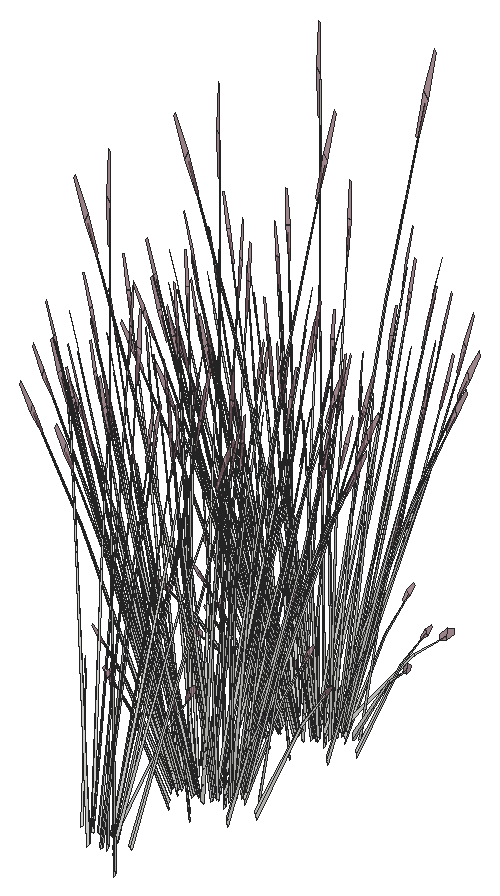
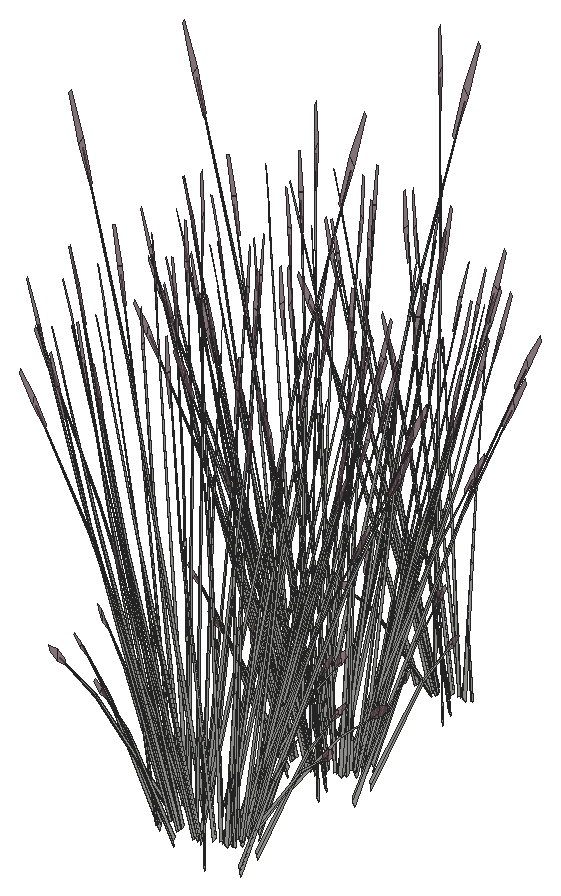
# SketchUp Ruby script. Lengths in inches.
U = 1.inch
M = Sketchup.active_model
def pt(a) = Geom::Point3d.new(a.map { |v| v * U })
def face(e, loops, mat)
  f = e.add_face(loops[0].map { |a| pt(a) })
  loops[1..].each { |l| e.add_face(l.map { |a| pt(a) }).erase! }
  f.material = f.back_material = mat if mat
  f
end
# faces: each face lists its corners as indices into pts; further lists are holes
def faces(e, pts, list, mat = nil) = list.each { |f| face(e, (f[0].is_a?(Array) ? f : [f]).map { |l| l.map { |i| pts[i] } }, mat) }
# xy, xz, yz: faces in a plane at the given z, y or x. An outline is a flat list of corners, or four numbers for a rectangle; further outlines are holes
def ring(l) = l.size == 4 ? [[l[0], l[1]], [l[2], l[1]], [l[2], l[3]], [l[0], l[3]]] : l.each_slice(2).to_a
def flat(e, list, mat, &to3) = list.each { |f| face(e, (f[0].is_a?(Array) ? f : [f]).map { |l| ring(l).map { |u, v| to3.(u, v) } }, mat) }
def xy(e, z, list, mat = nil) = flat(e, list, mat) { |x, y| [x, y, z] }
def xz(e, y, list, mat = nil) = flat(e, list, mat) { |x, z| [x, y, z] }
def yz(e, x, list, mat = nil) = flat(e, list, mat) { |y, z| [x, y, z] }
def lines(e, pts, list) = list.each { |a, b| e.add_line(pt(pts[a]), pt(pts[b])) }
# prism: a flat outline (further loops are holes) pulled along v
def prism(e, loops, v, mat = nil)
  f = face(e, loops, mat); d = Geom::Vector3d.new(v.map { |x| x * U })
  f.pushpull(f.normal.samedirection?(d) ? d.length : -d.length)
end
def box(e, o, s, mat = nil) = prism(e, [[o, [o[0] + s[0], o[1], o[2]], [o[0] + s[0], o[1] + s[1], o[2]], [o[0], o[1] + s[1], o[2]]]], [0, 0, s[2]], mat)
def at(x, y, z, deg = 0) = Geom::Transformation.translation(pt([x, y, z])) * Geom::Transformation.rotation(ORIGIN, Z_AXIS, deg.degrees)
def axes(o, x, y, z) = Geom::Transformation.new([*x, 0, *y, 0, *z, 0, *pt(o).to_a, 1])
def part(name) = M.definitions.add(name)
# library, detail: a bought-in or finely detailed component or shape, given as its bounding box
def library(name, o, s) = part(name).tap { |d| box(d.entities, o, s) }
def detail(e, o, s) = box(e.add_group.entities, o, s)
def put(e, d, t, mat = nil) = e.add_instance(d, t).tap { |i| i.material = mat if mat }
def group(e, t, mat = nil) = e.add_group.tap { |g| g.transformation = t; g.material = mat if mat }.entities
root = M.entities
M.materials.add("LightPink_Translucent").color = [144, 107, 117]
M.materials["LightPink_Translucent"].alpha = 0.75
c1 = part("blade")
p = [[2.15,0.21,22],[0,0.17,0],[0.09,0.45,0],[2.18,0.31,22],[2.29,0.31,22],[0.38,0.45,0],
  [2.48,0.24,33],[2.49,0.24,33],[2.48,0.22,33]]
faces(c1.entities,p,[[0,1,2,3],[4,5,2,3],[6,3,4,7],[8,0,3,6]])
c2 = part("seeds")
p = [[0.3,-0.1,1.38],[-0.01,-0.03,1.59],[-0.01,-0.03,0.03],[0.14,-0.07,-0.07],[0.29,-0.03,3],[0.15,0.01,3.11]]
faces(c2.entities,p,[[0,1,2,3],[1,0,4,5]],"LightPink_Translucent")
c3 = part("blade with seeds")
put(c3.entities,c1,at(0,0,0))
put(c3.entities,c2,axes([2.4,0.25,30.99],[1.5799,-0.05474,1.17369],[-0.12525,1.92788,0.29478],[-0.07173,-0.02425,1.56792]))
put(root,c3,axes([334.74,315.96,50.51],[-0.01379,-0.36791,1.24828],[0.62424,0.09537,0.52853],[-0.14764,0.20132,1.17828]))
put(root,c3,axes([334.79,317.375,52.14],[0.49824,-0.09289,-0.45151],[0.08716,0.35177,-0.34973],[0.13382,0.10081,0.86392]))
put(root,c3,axes([332.16,316.625,51.43],[0.09401,-0.13431,1.51428],[0.3944,0.27795,0.12244],[-0.17792,0.17323,0.64734]))
put(root,c3,axes([332.27,317.38,52],[-0.34164,0.20573,-0.31292],[-0.3234,-0.23491,0.40398],[-0.04921,0.11936,0.77298]))
put(root,c3,axes([331.09,317.32,52.17],[-0.01255,0.07733,1.54581],[0.35618,0.269,-0.24447],[-0.09325,0.12721,0.12397]))
put(root,c3,axes([333.25,317.55,52.45],[0.49409,-0.18193,-0.10745],[0.24281,0.32289,-0.59638],[0.06519,0.13607,0.90619]))
put(root,c3,axes([332.48,318.18,50.44],[-0.01307,-0.23234,1.01491],[0.32652,0.16572,0.74569],[-0.06422,0.11074,0.22354]))
put(root,c3,axes([332.61,317.28,52.42],[0.36145,0.26255,-0.50118],[-0.38183,0.22994,-0.3882],[-0.055,0.1334,0.95895]))
put(root,c3,axes([333.68,317.54,52.14],[0.49634,0.09796,-0.45151],[-0.17013,0.33585,-0.34973],[0.04551,0.13522,0.86392]))
put(root,c3,axes([333.96,316.85,51.43],[-0.11542,-0.12546,1.51428],[0.53333,-0.10562,0.12244],[0.12054,0.19696,0.64734]))
put(root,c3,axes([333.45,317.74,52],[-0.15222,0.30049,-0.31292],[-0.44409,-0.08764,0.40398],[0.04072,0.12098,0.77298]))
put(root,c3,axes([332.49,317.16,52.72],[-0.01314,0.36145,-0.69681],[-0.55324,-0.02428,0.08409],[-0.05838,0.15313,0.9857]))
put(root,c3,axes([333.02,316.91,51.43],[-0.01236,-0.14998,1.51428],[0.53562,0.09949,0.12244],[-0.03313,0.21373,0.64734]))
put(root,c3,axes([333.5,317.47,52.4],[0.24099,0.31773,-0.62776],[-0.49607,0.17707,0.07576],[0.05635,0.15352,0.88802]))
put(root,c3,axes([333.14,318.28,52.17],[0.064,0.06292,1.54581],[0.51651,0.02472,-0.24447],[0.05194,0.13877,0.12397]))
put(root,c3,axes([332.31,317.67,50.97],[0.01109,-0.20172,1.3638],[0.49896,0.10655,0.18846],[-0.04323,0.21498,0.64398]))
put(root,c3,axes([332.69,324.99,51.43],[0.11542,0.12546,1.51428],[-0.53333,0.10562,0.12244],[-0.12054,-0.19696,0.64734]))
put(root,c3,axes([334.11,325.08,52.4],[-0.24099,-0.31773,-0.62776],[0.49607,-0.17707,0.07576],[-0.05635,-0.15352,0.88802]))
put(root,c3,axes([335.12,325.39,52.4],[0.01314,-0.36145,-0.62776],[0.55324,0.02428,0.07576],[0.05838,-0.15313,0.88802]))
put(root,c3,axes([334.16,324.81,52],[0.15222,-0.30049,-0.31292],[0.44409,0.08764,0.40398],[-0.04072,-0.12098,0.77298]))
put(root,c3,axes([334.5,325.21,51.43],[-0.09401,0.13431,1.51428],[-0.3944,-0.27795,0.12244],[0.17792,-0.17323,0.64734]))
put(root,c3,axes([333.93,325.02,52.14],[-0.49634,-0.09796,-0.45151],[0.17013,-0.33585,-0.34973],[-0.04551,-0.13522,0.86392]))
put(root,c3,axes([334.24,324.18,50.44],[0.06477,0.22786,1.01491],[-0.35932,-0.1262,0.74569],[0.03867,-0.11667,0.22354]))
put(root,c3,axes([335.01,325.27,52.14],[-0.36145,-0.26255,-0.45151],[0.38183,-0.22994,-0.34973],[0.055,-0.1334,0.86392]))
put(root,c3,axes([334.36,325,52.45],[-0.49409,0.18193,-0.10745],[-0.24281,-0.32289,-0.59638],[-0.06519,-0.13607,0.90619]))
put(root,c3,axes([335.38,325.41,52.45],[-0.55492,-0.01936,-0.10745],[0.01517,-0.36657,-0.59638],[0.03855,-0.14118,0.90619]))
put(root,c3,axes([335.35,325.17,52],[0.34164,-0.20573,-0.31292],[0.3234,0.23491,0.40398],[0.04921,-0.11936,0.77298]))
put(root,c3,axes([332.39,324.45,50.44],[0.26338,0.136,1.01491],[-0.38358,0.08175,0.74569],[-0.08207,-0.10452,0.22354]))
put(root,c3,axes([333.03,325.17,52.4],[-0.43054,-0.18887,-0.62776],[0.30598,-0.33097,0.07576],[-0.15599,-0.11277,0.88802]))
put(root,c3,axes([332.88,324.92,52],[-0.07798,-0.31474,-0.31292],[0.44579,-0.08311,0.40398],[-0.11974,-0.09019,0.77298]))
put(root,c3,axes([331.92,325.38,51.43],[0.18755,0.06732,1.51428],[-0.38813,0.28243,0.12244],[-0.24191,-0.12741,0.64734]))
put(root,c3,axes([332.83,325.18,52.14],[-0.49824,0.09289,-0.45151],[-0.08716,-0.35177,-0.34973],[-0.13382,-0.10081,0.86392]))
put(root,c3,axes([335.77,326.02,52.4],[0.26374,-0.30832,-0.62776],[0.46217,0.21911,0.07576],[0.15748,-0.11171,0.88802]))
put(root,c3,axes([335.76,325.875,52.14],[-0.12971,-0.3568,-0.45151],[0.49122,-0.06241,-0.34973],[0.14077,-0.09583,0.86392]))
put(root,c3,axes([335.99,326.13,52.45],[-0.46706,-0.21546,-0.10745],[0.26908,-0.31203,-0.59638],[0.13196,-0.10846,0.90619]))
put(root,c3,axes([334.06,327.31,50.9375],[0.43633,0.15757,1.33654],[-0.42745,0.33945,0.52853],[-0.19146,-0.20119,1.12046]))
put(root,c3,axes([336.36,325.17,50.44],[-0.16818,0.19891,1.01491],[-0.14456,-0.26725,0.74569],[0.1389,-0.06697,0.22354]))
put(root,c3,axes([336.12,325.91,52],[0.43951,-0.05584,-0.31292],[0.11606,0.31924,0.40398],[0.12595,-0.08575,0.77298]))
put(root,c3,axes([331.85,325.47,52],[-0.28729,-0.24465,-0.31292],[0.32804,-0.23159,0.40398],[-0.16667,-0.03524,0.77298]))
put(root,c3,axes([332.15,325.64,52.4],[-0.50473,-0.00941,-0.62776],[0.0339,-0.39618,0.07576],[-0.21383,-0.04181,0.88802]))
put(root,c3,axes([331.98,325.72,52.14],[-0.36663,0.25884,-0.45151],[-0.32109,-0.27343,-0.34973],[-0.18628,-0.03938,0.86392]))
put(root,c3,axes([331.16,326.0625,50.44],[0.32236,-0.02796,1.01491],[-0.20448,0.24636,0.74569],[-0.1593,-0.03696,0.22354]))
put(root,c3,axes([332.18,325.45,52.45],[-0.02704,0.39739,-0.10745],[-0.51189,-0.01086,-0.59638],[-0.19715,-0.0276,0.90619]))
put(root,c3,axes([336.01,326.97,52.45],[-0.25405,-0.35383,-0.10745],[0.45089,-0.17388,-0.59638],[0.19001,-0.04668,0.90619]))
put(root,c3,axes([335.98,326.67,52.14],[0.13679,-0.35544,-0.45151],[0.46898,0.12183,-0.34973],[0.18882,-0.03259,0.86392]))
put(root,c3,axes([331.52,325.99,51.43],[0.20943,-0.00885,1.51428],[-0.13893,0.38357,0.12244],[-0.29846,-0.02372,0.64734]))
put(root,c3,axes([335.9,326.8,52.4],[0.44368,-0.17257,-0.62776],[0.24726,0.35524,0.07576],[0.21437,-0.04035,0.88802]))
put(root,c3,axes([336.27,326.83,52],[0.41962,0.10901,-0.31292],[-0.12239,0.31802,0.40398],[0.16894,-0.02916,0.77298]))
put(root,c3,axes([331.34,326.32,52],[-0.41962,-0.10901,-0.31292],[0.12239,-0.31802,0.40398],[-0.16894,0.02916,0.77298]))
put(root,c3,axes([335.13,326.4375,51.43],[-0.20943,0.00885,1.51428],[0.13893,-0.38357,0.12244],[0.29846,0.02372,0.64734]))
put(root,c3,axes([332.62,326.27,50.95],[0.14352,-0.05653,1.56454],[0.04949,0.39467,0.12244],[-0.31087,0.05237,0.55918]))
put(root,c3,axes([337.16,326.89,50.44],[-0.31197,0.06451,1.01491],[0.14684,-0.26661,0.74569],[0.1655,0.01824,0.22354]))
put(root,c3,axes([331.63,326.49,52.14],[-0.13679,0.35544,-0.45151],[-0.46898,-0.12183,-0.34973],[-0.18882,0.03259,0.86392]))
put(root,c3,axes([331.61,326.18,52.45],[0.25405,0.35383,-0.10745],[-0.45089,0.17388,-0.59638],[-0.19001,0.04668,0.90619]))
put(root,c3,axes([336.62,327.72,51.47],[-0.09664,-0.32847,-0.03085],[0.45676,-0.07551,-0.13989],[0.09538,0.02082,0.4614]))
put(root,c3,axes([335.4375,327.71,52.45],[0.02704,-0.39739,-0.10745],[0.51189,0.01086,-0.59638],[0.19715,0.0276,0.90619]))
put(root,c3,axes([331.61,326.67,51.43],[0.17519,-0.08265,1.51428],[0.14749,0.38193,0.12244],[-0.27504,0.08632,0.64734]))
put(root,c3,axes([335.46,327.52,52.4],[0.50473,0.00941,-0.62776],[-0.0339,0.39618,0.07576],[0.21383,0.04181,0.88802]))
put(root,c3,axes([330.7,328.01,50.44],[0.21042,-0.1771,1.01491],[0.08303,0.28036,0.74569],[-0.15207,0.0502,0.22354]))
put(root,c3,axes([335.77,327.68,52],[0.28729,0.24465,-0.31292],[-0.32804,0.23159,0.40398],[0.16667,0.03524,0.77298]))
put(root,c3,axes([331.49,327.24,52],[-0.43951,0.05584,-0.31292],[-0.11606,-0.31924,0.40398],[-0.12595,0.08575,0.77298]))
put(root,c3,axes([334.73,327.05,51.43],[-0.18755,-0.06732,1.51428],[0.38813,-0.28243,0.12244],[0.24191,0.12741,0.64734]))
put(root,c3,axes([334.77,326.17,51.95],[-0.4363,-0.20303,1.22187],[0.46069,-0.31611,0.5272],[0.14077,0.1905,1.18105]))
put(root,c3,axes([331.625,327.02,52.45],[0.46706,0.21546,-0.10745],[-0.26908,0.31203,-0.59638],[-0.13196,0.10846,0.90619]))
put(root,c3,axes([335.43,327.82,50.44],[-0.28429,-0.11236,1.01491],[0.36709,-0.11416,0.74569],[0.09901,0.0967,0.22354]))
put(root,c3,axes([334.43,328.14,52.45],[0.30087,-0.33447,-0.10745],[0.43572,0.19269,-0.59638],[0.15146,0.0945,0.90619]))
put(root,c3,axes([332.25,326.93,51.43],[0.12611,-0.12006,1.51428],[0.31843,0.32408,0.12244],[-0.2184,0.14759,0.64734]))
put(root,c3,axes([331.86,327.28,52.14],[0.12971,0.3568,-0.45151],[-0.49122,0.06241,-0.34973],[-0.14077,0.09583,0.86392]))
put(root,c3,axes([334.74,326.55,50.51],[-0.01379,-0.36791,1.24828],[0.62424,0.09537,0.52853],[-0.14764,0.20132,1.17828]))
put(root,c3,axes([334.79,327.97,52.14],[0.49824,-0.09289,-0.45151],[0.08716,0.35177,-0.34973],[0.13382,0.10081,0.86392]))
put(root,c3,axes([332.16,327.22,51.43],[0.09401,-0.13431,1.51428],[0.3944,0.27795,0.12244],[-0.17792,0.17323,0.64734]))
put(root,c3,axes([332.27,327.98,52],[-0.34164,0.20573,-0.31292],[-0.3234,-0.23491,0.40398],[-0.04921,0.11936,0.77298]))
put(root,c3,axes([333.25,328.15,52.45],[0.49409,-0.18193,-0.10745],[0.24281,0.32289,-0.59638],[0.06519,0.13607,0.90619]))
put(root,c3,axes([332.48,328.78,50.44],[-0.01307,-0.23234,1.01491],[0.32652,0.16572,0.74569],[-0.06422,0.11074,0.22354]))
put(root,c3,axes([332.61,327.88,52.42],[0.36145,0.26255,-0.50118],[-0.38183,0.22994,-0.3882],[-0.055,0.1334,0.95895]))
put(root,c3,axes([333.68,328.14,52.14],[0.49634,0.09796,-0.45151],[-0.17013,0.33585,-0.34973],[0.04551,0.13522,0.86392]))
put(root,c3,axes([333.96,327.44,51.43],[-0.11542,-0.12546,1.51428],[0.53333,-0.10562,0.12244],[0.12054,0.19696,0.64734]))
put(root,c3,axes([333.45,328.34,52],[-0.15222,0.30049,-0.31292],[-0.44409,-0.08764,0.40398],[0.04072,0.12098,0.77298]))
put(root,c3,axes([332.49,327.76,52.72],[-0.01314,0.36145,-0.69681],[-0.55324,-0.02428,0.08409],[-0.05838,0.15313,0.9857]))
put(root,c3,axes([333.02,327.51,51.43],[-0.01236,-0.14998,1.51428],[0.53562,0.09949,0.12244],[-0.03313,0.21373,0.64734]))
put(root,c3,axes([332.69,334.69,51.43],[0.11542,0.12546,1.51428],[-0.53333,0.10562,0.12244],[-0.12054,-0.19696,0.64734]))
put(root,c3,axes([333.5,328.07,52.4],[0.24099,0.31773,-0.62776],[-0.49607,0.17707,0.07576],[0.05635,0.15352,0.88802]))
put(root,c3,axes([333.57,333.86,52.17],[-0.07723,-0.05479,1.54581],[-0.51538,0.03473,-0.24447],[-0.08225,-0.13104,0.12397]))
put(root,c3,axes([334.11,334.78,52.4],[-0.24099,-0.31773,-0.62776],[0.49607,-0.17707,0.07576],[-0.05635,-0.15352,0.88802]))
put(root,c3,axes([335.12,335.1,52.4],[0.01314,-0.36145,-0.62776],[0.55324,0.02428,0.07576],[0.05838,-0.15313,0.88802]))
put(root,c3,axes([332.31,328.27,50.97],[0.01109,-0.20172,1.3638],[0.49896,0.10655,0.18846],[-0.04323,0.21498,0.64398]))
put(root,c3,axes([335.89,334.53,52.17],[-0.00487,-0.07777,1.54581],[-0.41166,-0.22476,-0.24447],[0.06364,-0.13625,0.12397]))
put(root,c3,axes([334.16,334.51,52],[0.15222,-0.30049,-0.31292],[0.44409,0.08764,0.40398],[-0.04072,-0.12098,0.77298]))
put(root,c3,axes([334.5,334.91,51.43],[-0.09401,0.13431,1.51428],[-0.3944,-0.27795,0.12244],[0.17792,-0.17323,0.64734]))
put(root,c3,axes([333.93,334.72,52.14],[-0.49634,-0.09796,-0.45151],[0.17013,-0.33585,-0.34973],[-0.04551,-0.13522,0.86392]))
put(root,c3,axes([334.24,333.88,50.44],[0.06477,0.22786,1.01491],[-0.35932,-0.1262,0.74569],[0.03867,-0.11667,0.22354]))
put(root,c3,axes([335.01,334.98,52.14],[-0.36145,-0.26255,-0.45151],[0.38183,-0.22994,-0.34973],[0.055,-0.1334,0.86392]))
put(root,c3,axes([334.36,334.7,52.45],[-0.49409,0.18193,-0.10745],[-0.24281,-0.32289,-0.59638],[-0.06519,-0.13607,0.90619]))
put(root,c3,axes([335.38,335.11,52.45],[-0.55492,-0.01936,-0.10745],[0.01517,-0.36657,-0.59638],[0.03855,-0.14118,0.90619]))
put(root,c3,axes([335.35,334.88,52],[0.34164,-0.20573,-0.31292],[0.3234,0.23491,0.40398],[0.04921,-0.11936,0.77298]))
put(root,c3,axes([332.39,334.15,50.44],[0.26338,0.136,1.01491],[-0.38358,0.08175,0.74569],[-0.08207,-0.10452,0.22354]))
put(root,c3,axes([333.03,334.875,52.4],[-0.43054,-0.18887,-0.62776],[0.30598,-0.33097,0.07576],[-0.15599,-0.11277,0.88802]))
put(root,c3,axes([332.88,334.625,52],[-0.07798,-0.31474,-0.31292],[0.44579,-0.08311,0.40398],[-0.11974,-0.09019,0.77298]))
put(root,c3,axes([331.92,335.08,51.43],[0.18755,0.06732,1.51428],[-0.38813,0.28243,0.12244],[-0.24191,-0.12741,0.64734]))
put(root,c3,axes([332.83,334.88,52.14],[-0.49824,0.09289,-0.45151],[-0.08716,-0.35177,-0.34973],[-0.13382,-0.10081,0.86392]))
put(root,c3,axes([335.77,335.72,52.4],[0.26374,-0.30832,-0.62776],[0.46217,0.21911,0.07576],[0.15748,-0.11171,0.88802]))
put(root,c3,axes([335.76,335.58,52.14],[-0.12971,-0.3568,-0.45151],[0.49122,-0.06241,-0.34973],[0.14077,-0.09583,0.86392]))
put(root,c3,axes([331.88,334.46,52.17],[-0.10864,-0.00276,1.54581],[-0.34587,0.27582,-0.24447],[-0.18454,-0.05636,0.12397]))
put(root,c3,axes([335.99,335.84,52.45],[-0.46706,-0.21546,-0.10745],[0.26908,-0.31203,-0.59638],[0.13196,-0.10846,0.90619]))
put(root,c3,axes([334.06,337.01,50.9375],[0.43633,0.15757,1.33654],[-0.42745,0.33945,0.52853],[-0.19146,-0.20119,1.12046]))
put(root,c3,axes([336.36,334.87,50.44],[-0.16818,0.19891,1.01491],[-0.14456,-0.26725,0.74569],[0.1389,-0.06697,0.22354]))
put(root,c3,axes([336.12,335.62,52],[0.43951,-0.05584,-0.31292],[0.11606,0.31924,0.40398],[0.12595,-0.08575,0.77298]))
put(root,c3,axes([331.85,335.18,52],[-0.28729,-0.24465,-0.31292],[0.32804,-0.23159,0.40398],[-0.16667,-0.03524,0.77298]))
put(root,c3,axes([332.15,335.34,52.4],[-0.50473,-0.00941,-0.62776],[0.0339,-0.39618,0.07576],[-0.21383,-0.04181,0.88802]))
put(root,c3,axes([337.39,336.12,52.17],[0.07006,-0.05952,1.54581],[-0.08968,-0.3651,-0.24447],[0.1758,-0.06922,0.12397]))
put(root,c3,axes([331.98,335.42,52.14],[-0.36663,0.25884,-0.45151],[-0.32109,-0.27343,-0.34973],[-0.18628,-0.03938,0.86392]))
put(root,c3,axes([331.16,335.77,50.44],[0.32236,-0.02796,1.01491],[-0.20448,0.24636,0.74569],[-0.1593,-0.03696,0.22354]))
put(root,c3,axes([332.18,335.15,52.45],[-0.02704,0.39739,-0.10745],[-0.51189,-0.01086,-0.59638],[-0.19715,-0.0276,0.90619]))
put(root,c3,axes([336.01,336.68,52.45],[-0.25405,-0.35383,-0.10745],[0.45089,-0.17388,-0.59638],[0.19001,-0.04668,0.90619]))
put(root,c3,axes([335.98,336.37,52.14],[0.13679,-0.35544,-0.45151],[0.46898,0.12183,-0.34973],[0.18882,-0.03259,0.86392]))
put(root,c3,axes([331.52,335.7,51.43],[0.20943,-0.00885,1.51428],[-0.13893,0.38357,0.12244],[-0.29846,-0.02372,0.64734]))
put(root,c3,axes([335.9,336.5,52.4],[0.44368,-0.17257,-0.62776],[0.24726,0.35524,0.07576],[0.21437,-0.04035,0.88802]))
put(root,c3,axes([336.27,336.53,52],[0.41962,0.10901,-0.31292],[-0.12239,0.31802,0.40398],[0.16894,-0.02916,0.77298]))
put(root,c3,axes([331.34,336.03,52],[-0.41962,-0.10901,-0.31292],[0.12239,-0.31802,0.40398],[-0.16894,0.02916,0.77298]))
put(root,c3,axes([335.13,336.14,51.43],[-0.20943,0.00885,1.51428],[0.13893,-0.38357,0.12244],[0.29846,0.02372,0.64734]))
put(root,c3,axes([332.62,335.97,50.95],[0.14352,-0.05653,1.56454],[0.04949,0.39467,0.12244],[-0.31087,0.05237,0.55918]))
put(root,c3,axes([337.16,336.6,50.44],[-0.31197,0.06451,1.01491],[0.14684,-0.26661,0.74569],[0.1655,0.01824,0.22354]))
put(root,c3,axes([331.08,336.24,52.17],[-0.08245,0.05073,1.54581],[0.00701,0.37067,-0.24447],[-0.18899,0.0482,0.12397]))
put(root,c3,axes([331.63,336.19,52.14],[-0.13679,0.35544,-0.45151],[-0.46898,-0.12183,-0.34973],[-0.18882,0.03259,0.86392]))
put(root,c3,axes([331.61,335.89,52.45],[0.25405,0.35383,-0.10745],[-0.45089,0.17388,-0.59638],[-0.19001,0.04668,0.90619]))
put(root,c3,axes([336.62,337.42,51.47],[-0.09664,-0.32847,-0.03085],[0.45676,-0.07551,-0.13989],[0.09538,0.02082,0.4614]))
put(root,c3,axes([335.4375,337.41,52.45],[0.02704,-0.39739,-0.10745],[0.51189,0.01086,-0.59638],[0.19715,0.0276,0.90619]))
put(root,c3,axes([335.88,337.17,52.17],[0.10831,-0.00661,1.54581],[0.29709,-0.30358,-0.24447],[0.19266,0.04007,0.12397]))
put(root,c3,axes([331.61,336.375,51.43],[0.17519,-0.08265,1.51428],[0.14749,0.38193,0.12244],[-0.27504,0.08632,0.64734]))
put(root,c3,axes([335.46,337.22,52.4],[0.50473,0.00941,-0.62776],[-0.0339,0.39618,0.07576],[0.21383,0.04181,0.88802]))
put(root,c3,axes([330.7,337.71,50.44],[0.21042,-0.1771,1.01491],[0.08303,0.28036,0.74569],[-0.15207,0.0502,0.22354]))
put(root,c3,axes([335.77,337.38,52],[0.28729,0.24465,-0.31292],[-0.32804,0.23159,0.40398],[0.16667,0.03524,0.77298]))
put(root,c3,axes([331.49,336.94,52],[-0.43951,0.05584,-0.31292],[-0.11606,-0.31924,0.40398],[-0.12595,0.08575,0.77298]))
put(root,c3,axes([334.73,336.76,51.43],[-0.18755,-0.06732,1.51428],[0.38813,-0.28243,0.12244],[0.24191,0.12741,0.64734]))
put(root,c3,axes([334.77,335.87,51.95],[-0.4363,-0.20303,1.22187],[0.46069,-0.31611,0.5272],[0.14077,0.1905,1.18105]))
put(root,c3,axes([331.625,336.73,52.45],[0.46706,0.21546,-0.10745],[-0.26908,0.31203,-0.59638],[-0.13196,0.10846,0.90619]))
put(root,c3,axes([335.43,337.52,50.44],[-0.28429,-0.11236,1.01491],[0.36709,-0.11416,0.74569],[0.09901,0.0967,0.22354]))
put(root,c3,axes([334.43,337.84,52.45],[0.30087,-0.33447,-0.10745],[0.43572,0.19269,-0.59638],[0.15146,0.0945,0.90619]))
put(root,c3,axes([332.25,336.63,51.43],[0.12611,-0.12006,1.51428],[0.31843,0.32408,0.12244],[-0.2184,0.14759,0.64734]))
put(root,c3,axes([331.86,336.98,52.14],[0.12971,0.3568,-0.45151],[-0.49122,0.06241,-0.34973],[-0.14077,0.09583,0.86392]))
put(root,c3,axes([334.74,336.26,50.51],[-0.01379,-0.36791,1.24828],[0.62424,0.09537,0.52853],[-0.14764,0.20132,1.17828]))
put(root,c3,axes([334.79,337.68,52.14],[0.49824,-0.09289,-0.45151],[0.08716,0.35177,-0.34973],[0.13382,0.10081,0.86392]))
put(root,c3,axes([332.16,336.93,51.43],[0.09401,-0.13431,1.51428],[0.3944,0.27795,0.12244],[-0.17792,0.17323,0.64734]))
put(root,c3,axes([332.27,337.68,52],[-0.34164,0.20573,-0.31292],[-0.3234,-0.23491,0.40398],[-0.04921,0.11936,0.77298]))
put(root,c3,axes([331.09,337.62,52.17],[-0.01255,0.07733,1.54581],[0.35618,0.269,-0.24447],[-0.09325,0.12721,0.12397]))
put(root,c3,axes([333.25,337.86,52.45],[0.49409,-0.18193,-0.10745],[0.24281,0.32289,-0.59638],[0.06519,0.13607,0.90619]))
put(root,c3,axes([332.48,338.48,50.44],[-0.01307,-0.23234,1.01491],[0.32652,0.16572,0.74569],[-0.06422,0.11074,0.22354]))
put(root,c3,axes([332.61,337.59,52.42],[0.36145,0.26255,-0.50118],[-0.38183,0.22994,-0.3882],[-0.055,0.1334,0.95895]))
put(root,c3,axes([333.68,337.84,52.14],[0.49634,0.09796,-0.45151],[-0.17013,0.33585,-0.34973],[0.04551,0.13522,0.86392]))
